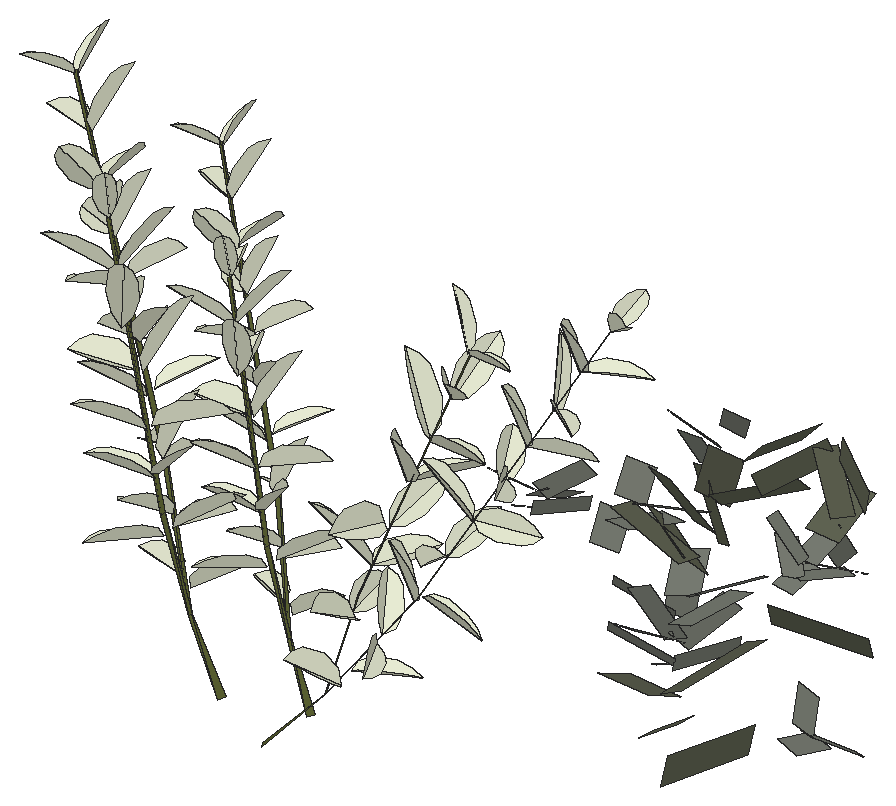
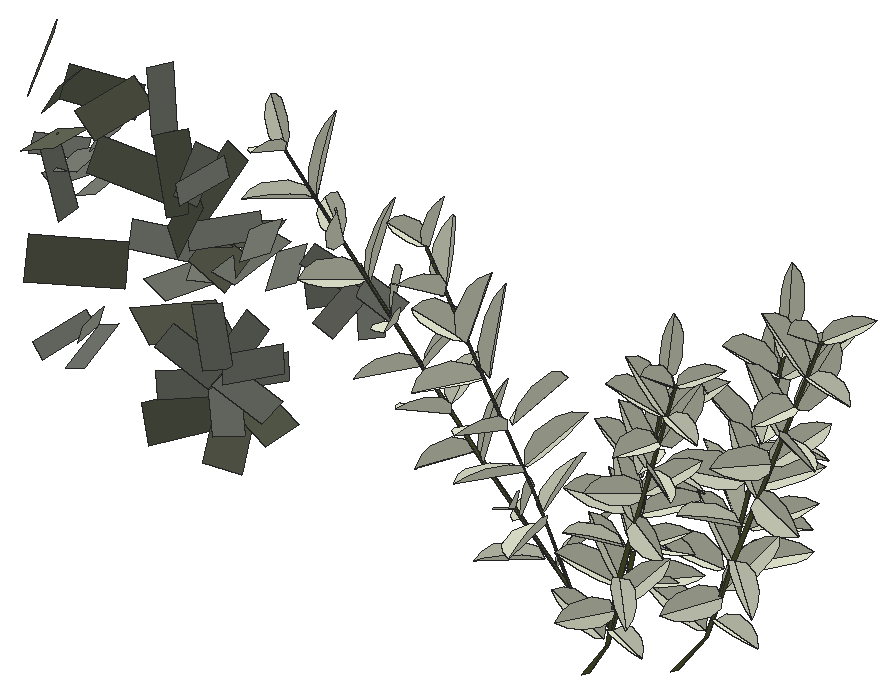
# SketchUp Ruby script. Lengths in inches.
U = 1.inch
M = Sketchup.active_model
def pt(a) = Geom::Point3d.new(a.map { |v| v * U })
def face(e, loops, mat)
  f = e.add_face(loops[0].map { |a| pt(a) })
  loops[1..].each { |l| e.add_face(l.map { |a| pt(a) }).erase! }
  f.material = f.back_material = mat if mat
  f
end
# faces: each face lists its corners as indices into pts; further lists are holes
def faces(e, pts, list, mat = nil) = list.each { |f| face(e, (f[0].is_a?(Array) ? f : [f]).map { |l| l.map { |i| pts[i] } }, mat) }
# xy, xz, yz: faces in a plane at the given z, y or x. An outline is a flat list of corners, or four numbers for a rectangle; further outlines are holes
def ring(l) = l.size == 4 ? [[l[0], l[1]], [l[2], l[1]], [l[2], l[3]], [l[0], l[3]]] : l.each_slice(2).to_a
def flat(e, list, mat, &to3) = list.each { |f| face(e, (f[0].is_a?(Array) ? f : [f]).map { |l| ring(l).map { |u, v| to3.(u, v) } }, mat) }
def xy(e, z, list, mat = nil) = flat(e, list, mat) { |x, y| [x, y, z] }
def xz(e, y, list, mat = nil) = flat(e, list, mat) { |x, z| [x, y, z] }
def yz(e, x, list, mat = nil) = flat(e, list, mat) { |y, z| [x, y, z] }
def lines(e, pts, list) = list.each { |a, b| e.add_line(pt(pts[a]), pt(pts[b])) }
# prism: a flat outline (further loops are holes) pulled along v
def prism(e, loops, v, mat = nil)
  f = face(e, loops, mat); d = Geom::Vector3d.new(v.map { |x| x * U })
  f.pushpull(f.normal.samedirection?(d) ? d.length : -d.length)
end
def box(e, o, s, mat = nil) = prism(e, [[o, [o[0] + s[0], o[1], o[2]], [o[0] + s[0], o[1] + s[1], o[2]], [o[0], o[1] + s[1], o[2]]]], [0, 0, s[2]], mat)
def at(x, y, z, deg = 0) = Geom::Transformation.translation(pt([x, y, z])) * Geom::Transformation.rotation(ORIGIN, Z_AXIS, deg.degrees)
def axes(o, x, y, z) = Geom::Transformation.new([*x, 0, *y, 0, *z, 0, *pt(o).to_a, 1])
def part(name) = M.definitions.add(name)
# library, detail: a bought-in or finely detailed component or shape, given as its bounding box
def library(name, o, s) = part(name).tap { |d| box(d.entities, o, s) }
def detail(e, o, s) = box(e.add_group.entities, o, s)
def put(e, d, t, mat = nil) = e.add_instance(d, t).tap { |i| i.material = mat if mat }
def group(e, t, mat = nil) = e.add_group.tap { |g| g.transformation = t; g.material = mat if mat }.entities
root = M.entities
M.materials.add("asdfasdf0165f6asdLeafVar1sfd015as60f1as6").color = [231, 235, 211]
M.materials.add("dw_stemssadfasdfa0sdf1s01d6w1").color = [90, 97, 50]
M.materials.add("viburnumblaasdfas0df1w06d").color = [98, 102, 84]
M.materials.add("viburnumbladsadfasdfad0w122").color = [125, 129, 119]
c1 = part("Component\#314")
p = [[0.14,0,0],[2.58,0.05,0.25],[2.44,5.11,2.64],[0,5.05,2.39]]
faces(c1.entities,p,[[0,1,2,3]],"viburnumblaasdfas0df1w06d")
c2 = part("viburnumblad1\#2")
put(c2.entities,c1,axes([-37.25,6.23,19.31],[75.98784,0,0],[0,65.50676,0],[0,0,75.98784]))
c3 = part("Component\#315")
p = [[0.25,0,0],[2.05,0.01,0.35],[1.81,4.2,1.66],[0,4.19,1.3125]]
faces(c3.entities,p,[[0,1,2,3]],"viburnumbladsadfasdfad0w122")
c4 = part("viburnumblad2")
put(c4.entities,c3,axes([-19.23,-4.49,-32.18],[83.35428,0,0],[0,79.38502,0],[0,0,83.35428]))
c5 = part("vdw_leaf\#3")
p = [[0,0,0],[-2.77,1.61,2.32],[-4.3125,6.1,4.5],[-3.97,13.49,6.09],[-2.47,18.57,6.3],[-0.2,22.73,5.75],
  [2.54,19.66,6.85],[4.3,15.93,7.09],[5.03,7.6,5.43],[3.32,1.76,2.74]]
faces(c5.entities,p,[[0,1,2,3,4,5],[0,5,6,7,8,9]],"asdfasdf0165f6asdLeafVar1sfd015as60f1as6")
c6 = part("dw_brancj_2\#2")
p = [[9.7,-0.22,29.95],[0.23,-1.96,0.34],[-0.05,1.51,0.11],[9.65,1.51,29.46],[18.64,-8.75,84.43],[18.96,-6.63,84.625],
  [1.53,6.02,63.68],[1.42,8.18,63.25],[-10.58,8.77,161.17],[-10.41,9.98,160.68],[26.34,-9.37,211.72],[26.57,-8.28,211.23]]
faces(c6.entities,p,[[0,1,2],[0,2,3],[4,0,3],[4,3,5],[6,0,3],[6,3,7],[8,6,7],[8,7,9],
  [10,4,5],[10,5,11]],"dw_stemssadfasdfa0sdf1s01d6w1")
c7 = part("vdw_branch2\#3")
put(c7.entities,c5,axes([19.53,-5.9,102.42],[1.12377,-0.50004,0],[0.46097,1.03596,0.47664],[-0.19377,-0.43548,1.13389]))
put(c7.entities,c5,axes([-5.89,6.52,109.44],[-1.07209,0.83679,0],[-0.77141,-0.98832,0.52702],[0.32427,0.41545,1.25373]))
put(c7.entities,c5,axes([-0.44,8.23,75.28],[0.88709,-0.9947,0],[0.92159,0.82189,0.33087],[-0.25219,-0.22491,1.26111]))
put(c7.entities,c5,axes([24.71,-8.97,190.81],[-0.82641,0.91101,0],[-0.83983,-0.76184,0.47664],[0.35303,0.32025,1.13389]))
put(c7.entities,c5,axes([-2.29,8.24,91.35],[1.24603,-0.47303,0],[0.43826,1.15445,0.33087],[-0.11993,-0.31592,1.26111]))
put(c7.entities,c5,axes([12.26,-3.11,37.92],[-0.64625,1.02205,0.22511],[-1.04383,-0.61044,-0.22511],[-0.07533,-0.30931,1.18809]))
put(c7.entities,c5,axes([26.17,-9.17,210.27],[-0.99452,-0.10453,0],[0.09636,-0.91681,0.38752],[-0.04051,0.38539,0.92186]))
put(c7.entities,c5,axes([-6.07,9.4,125.35],[-0.90214,-0.98107,0],[0.90896,-0.83583,0.33087],[-0.24874,0.22873,1.26111]))
put(c7.entities,c5,axes([-4.13,7.29,110.58],[0.44715,-1.078,0.64369],[1.05816,0.63649,0.33087],[-0.58725,0.40856,1.09216]))
put(c7.entities,c5,axes([23.91,-8.22,171.96],[0.62307,0.85009,-0.63406],[-0.71531,0.8798,0.47664],[0.78296,0.12729,0.94004]))
put(c7.entities,c6,at(-0.09,0.18,-0.25),"dw_stemssadfasdfa0sdf1s01d6w1")
put(c7.entities,c5,axes([23.34,-9.65,156.59],[-0.31364,-1.00782,0.58216],[1.10369,-0.17062,0.29925],[-0.17137,0.6239,0.98776]))
put(c7.entities,c5,axes([15.03,-3.37,58.83],[-1.05425,-0.00194,0.58442],[-0.14303,-1.11707,-0.26172],[0.55355,-0.3046,0.99755]))
put(c7.entities,c5,axes([-11.625,9.46,160.37],[0.36812,0.92978,0],[-0.85713,0.33936,0.38752],[0.3603,-0.14265,0.92186]))
put(c7.entities,c5,axes([21.32,-8.53,138.72],[1.21379,0.19904,0],[-0.19904,1.21379,0],[0,0,1.23]))
put(c7.entities,c5,axes([22.54,-9.2,141.43],[-1.02887,0.17955,0.60182],[-0.23387,-1.13057,-0.06253],[0.56696,-0.17376,1.02111]))
put(c7.entities,c5,axes([23.9,-8.82,173.84],[-1.14567,-0.37474,0],[0.35918,-1.0981,0.04438],[-0.01409,0.04308,1.17993]))
put(c7.entities,c5,axes([-7.84,8.92,143.59],[-1.26971,0.40522,0],[-0.37543,-1.17638,0.33087],[0.10274,0.32192,1.26111]))
put(c7.entities,c5,axes([19.77,-8.01,85.98],[-0.32405,-1.14591,0.18674],[1.10278,-0.32969,-0.10948],[0.15845,0.14442,1.16117]))
put(c7.entities,c5,axes([-0.62,5.76,76.34],[-0.08879,1.17576,-0.67771],[-1.34525,-0.16582,-0.11144],[-0.17897,0.66309,1.17383]))
put(c7.entities,c5,axes([20.49,-8.22,121.07],[0.39924,-0.78471,-0.8233],[1.08735,0.33121,0.2116],[0.09035,-0.83005,0.83495]))
put(c7.entities,c5,axes([15.15,-3.72,62.9],[1.16251,0.40128,-0.0211],[-0.39924,1.16074,0.07874],[0.0456,-0.06757,1.2273]))
put(c7.entities,c5,axes([20.72,-8.08,120.26],[-0.03693,1.2277,-0.06551],[-1.22944,-0.03698,0],[-0.00197,0.06548,1.22825]))
put(c7.entities,c5,axes([22.58,-8.36,155.57],[-0.56247,1.09386,0],[-1.00839,-0.51852,0.47664],[0.42389,0.21796,1.13389]))
put(c7.entities,c5,axes([3.97,3.13,57.96],[-1.09459,0.76041,0],[-0.72262,-1.0402,-0.1735],[-0.10109,-0.14552,1.29352]))
put(c7.entities,c5,axes([-10.8,9.06,160.75],[-0.66334,-0.72138,0],[0.66835,-0.61458,0.24329],[-0.1829,0.16818,0.92729]))
put(c7.entities,c5,axes([19.06,-9.3125,103.96],[-1.01345,0.25553,-0.60051],[-0.2265,-1.12952,-0.09839],[-0.59598,0.03076,1.01889]))
put(c7.entities,c5,axes([18.07,-6.2,81.7],[-0.56247,1.09386,0],[-1.00839,-0.51852,0.47664],[0.42389,0.21796,1.13389]))
put(c7.entities,c5,axes([12.95,-0.39,43.31],[0.13044,-1.19832,0],[1.11025,0.12085,0.29925],[-0.30382,-0.03307,1.14057]))
put(c7.entities,c5,axes([2.28,8.28,56.18],[1.32413,-0.31027,0],[0.30923,1.31968,-0.11144],[0.02542,0.1085,1.35543]))
put(c7.entities,c5,axes([-7.55,9.96,143.07],[1.34251,-0.21744,0],[0.20045,1.23761,0.52702],[-0.08426,-0.52024,1.25373]))
put(c7.entities,c5,axes([26.15,-8.25,210.66],[0.94661,-0.25364,0],[0.235,0.87703,0.24329],[-0.06431,-0.24,0.92729]))
put(c7.entities,c5,axes([-6.48,11.37,125.16],[0.64635,1.10315,0.46356],[-1.16569,0.46153,0.52702],[0.27017,-0.6478,1.16488]))
put(c7.entities,c5,axes([25.74,-8.35,191.28],[0.13044,-1.19832,0],[1.11025,0.12085,0.29925],[-0.30382,-0.03307,1.14057]))
put(c7.entities,c5,axes([-5.125,7.47,91.6],[-1.10024,0.63688,0.48318],[-0.78682,-1.00808,-0.46292],[0.14137,-0.65404,1.184]))
put(root,c2,axes([1229.8,292.03,5.5],[0.00521,-0.00318,0.0136],[0.01189,0.01244,-0.00164],[-0.00949,0.00985,0.00593]))
put(root,c4,axes([1238.96,294.58,23.71],[-0.00315,0.00923,-0.0035],[-0.009,-0.00109,0.00491],[0.00408,0.00455,0.00739]))
put(root,c2,axes([1229.78,294.23,20.15],[-0.00128,0.01292,-0.00526],[-0.01614,-0.0018,-0.00049],[-0.00098,0.00473,0.0118]))
put(root,c2,axes([1229.76,292.29,11.59],[0.01313,-0.00582,0.00636],[0.00841,0.01593,-0.00278],[-0.00467,0.00494,0.01417]))
put(root,c4,axes([1223.64,293.02,20.79],[0.00973,0.00497,-0.00674],[-0.00836,0.01112,-0.00387],[0.00402,0.00678,0.0108]))
put(root,c7,axes([1195,291.84,-0.375],[-0.13136,0.05263,-0.10053],[-0.06077,-0.15168,0],[-0.07584,0.03038,0.17413]))
put(root,c4,axes([1216.74,293.95,20.41],[0.00898,0.00541,-0.00233],[-0.00533,0.00547,-0.00762],[-0.00249,0.00719,0.00626]))
put(root,c2,axes([1230.42,296.33,21.7],[-0.01202,0.00402,-0.00269],[-0.00561,-0.01134,0.00795],[0.00019,0.00723,0.00942]))
put(root,c7,axes([1199.63,290.12,-1.28],[0.12089,0.06455,-0.10951],[-0.07696,0.14414,0],[0.0785,0.04192,0.16863]))
put(root,c4,axes([1216.89,294.82,21.52],[0.00286,0.007,-0.00749],[-0.01015,0.00031,-0.00351],[-0.0019,0.00782,0.00576]))
put(root,c4,axes([1238.02,294.15,22.79],[0.00444,0.00768,-0.00528],[-0.00777,0.00538,0.00119],[0.00402,0.0037,0.00783]))
put(root,c2,axes([1227.75,293.87,10.14],[0.00536,0.01158,-0.00521],[-0.01304,0.00197,-0.00903],[-0.0059,0.00728,0.01011]))
put(root,c4,axes([1229.72,295.18,18.16],[0.00715,-0.01146,0.00475],[0.01219,0.00751,-0.00024],[-0.0023,0.00416,0.01351]))
put(root,c4,axes([1217.29,294.85,19.55],[0.00494,-0.0045,0.00826],[0.00853,0.00632,-0.00167],[-0.00419,0.00708,0.00554]))
put(root,c2,axes([1227.99,292.7,7.87],[0.01075,0.00741,0.00439],[-0.00265,0.0107,-0.01157],[-0.00831,0.00706,0.00843]))
put(root,c4,axes([1229.23,293.68,16.72],[0.01381,-0.0032,0.00202],[0.00375,0.01421,-0.00318],[-0.00124,0.00342,0.01385]))
put(root,c4,axes([1227.42,296.46,12.26],[-0.00484,0.0048,-0.00995],[-0.01148,-0.00686,0.00228],[-0.0044,0.00962,0.00678]))
put(root,c4,axes([1237.17,294.3,21.79],[0.00829,0.00118,-0.00446],[-0.00277,0.00969,-0.0025],[0.00431,0.00339,0.00782]))
put(root,c4,axes([1238.6875,296.25,22.97],[0.00315,-0.00923,0.0035],[0.00972,0.00216,-0.00297],[0.00178,0.00415,0.00836]))
put(root,c4,axes([1237.5,294.51,10.76],[0.00948,-0.00167,-0.00544],[-0.00216,0.00929,-0.00661],[0.00531,0.00641,0.00728]))
put(root,c4,axes([1217.69,296.07,20.33],[-0.00286,-0.007,0.00749],[0.00939,0.00159,0.0048],[-0.00429,0.00766,0.00474]))
put(root,c4,axes([1228.96,293.63,18.7],[0.01238,0.00695,-0.00189],[-0.0072,0.01199,-0.00308],[0.00008,0.00361,0.01386]))
put(root,c4,axes([1237.59,295.47,22.32],[0.00889,-0.00537,-0.00033],[0.00481,0.00824,-0.00432],[0.00239,0.00342,0.00851]))
put(root,c4,axes([1223.65,294.65,21.63],[0.01295,-0.00298,-0.00152],[0.00183,0.01176,-0.00745],[0.00286,0.00667,0.01124]))
put(root,c4,axes([1238.18,296,10.96],[0.0086,-0.00684,0.0012],[0.00538,0.00535,-0.00804],[0.0044,0.00684,0.00749]))
put(root,c4,axes([1238.31,295.04,11.96],[0.0048,0.00448,-0.0089],[-0.00793,0.0077,-0.0004],[0.00603,0.00655,0.00655]))
put(root,c2,axes([1235.11,295.17,26.65],[0.00085,-0.00676,0.01003],[0.01236,0.00601,0.00299],[-0.00572,0.00864,0.0063]))
put(root,c4,axes([1227.2,297.95,13],[-0.01065,-0.00175,-0.00643],[-0.00418,-0.00769,0.00902],[-0.00519,0.00978,0.00593]))
put(root,c4,axes([1224.45,296.34,22.32],[0.00818,-0.0094,0.00487],[0.01043,0.00611,-0.00572],[0.00179,0.0073,0.01107]))
put(root,c4,axes([1231.33,298.72,28.41],[-0.00994,-0.00547,0.00222],[0.00636,-0.00933,0.00551],[-0.00082,0.00596,0.01103]))
put(root,c2,axes([1241.92,297.13,26.98],[-0.00677,0.00906,0.00107],[-0.00671,-0.00636,0.00903],[0.00707,0.00408,0.0069]))
put(root,c2,axes([1229.54,294.79,20.07],[0.00337,0.00858,-0.01052],[-0.01574,0.00327,-0.00237],[0.0008,0.00999,0.00793]))
put(root,c4,axes([1216.47,295.5,20.44],[0.00984,0.00064,0.00419],[0.00246,0.0079,-0.00679],[-0.00344,0.00689,0.00616]))
put(root,c4,axes([1237.94,295.41,23.64],[0.00943,0.00164,-0.00397],[-0.00277,0.00969,-0.0025],[0.00332,0.00323,0.0083]))
put(root,c4,axes([1224,295.12,23.4],[0.01014,0.00518,-0.00703],[-0.00774,0.0103,-0.00358],[0.00402,0.00678,0.0108]))
put(root,c2,axes([1229.72,298.37,22.52],[-0.01137,-0.00525,0.00325],[0.00699,-0.00886,0.00961],[-0.00151,0.00884,0.00798]))
put(root,c2,axes([1240.32,296.03,26.31],[0.00134,0.01062,-0.0039],[-0.01115,0.00362,0.00577],[0.00594,0.00252,0.00833]))
put(root,c4,axes([1226.03,297.13,13.03],[0.00352,0.00882,-0.00823],[-0.01182,-0.0007,-0.00581],[-0.00432,0.00892,0.00772]))
put(root,c4,axes([1225.88,298.38,14.25],[-0.00504,0.005,-0.01036],[-0.01063,-0.00635,0.00211],[-0.0044,0.00962,0.00678]))
put(root,c2,axes([1230.89,297.1,20.58],[-0.00982,0.00575,-0.00616],[-0.00925,-0.00382,0.01097],[0.00277,0.01054,0.00496]))
put(root,c4,axes([1226.09,296.36,11.375],[0.01046,0.00781,-0.00132],[-0.00513,0.00543,-0.00849],[-0.00501,0.0081,0.0082]))
put(root,c2,axes([1233.82,297.51,16.09],[0.0041,-0.00986,0.01208],[0.01717,-0.00172,-0.00723],[0.00492,0.01267,0.00868]))
put(root,c4,axes([1229.02,299.35,25.03],[-0.01201,-0.00131,-0.00224],[-0.00042,-0.0083,0.00649],[-0.00262,0.00705,0.00788]))
put(root,c2,axes([1230.02,297.41,23.09],[0.00221,-0.01095,0.00807],[0.01572,0.00285,-0.00044],[-0.00114,0.008,0.01116]))
put(root,c2,axes([1233.66,295.63,28.32],[0.00897,-0.0006,0.00814],[0.00562,0.01175,-0.00532],[-0.00657,0.00665,0.00773]))
put(root,c4,axes([1226.56,297.39,10.64],[0.00529,-0.00535,0.00878],[0.00925,0.00849,-0.00041],[-0.00626,0.00721,0.00817]))
put(root,c4,axes([1226.55,299.51,13.37],[-0.01002,-0.00748,0.00127],[0.00432,-0.00389,0.01114],[-0.00624,0.00932,0.00567]))
put(root,c2,axes([1238.4375,295.95,24.83],[0.01113,0.00289,-0.00438],[-0.00454,0.01328,-0.00273],[0.00348,0.00335,0.01016]))
put(root,c4,axes([1237.75,300.29,20.6],[-0.0106,-0.00225,0.00809],[0.00771,-0.01018,0.00728],[0.00487,0.01032,0.00927]))
put(root,c4,axes([1226.75,298.72,11.66],[-0.00352,-0.00882,0.00823],[0.00998,0.00284,0.00731],[-0.00692,0.00849,0.00615]))
put(root,c7,axes([1199.9,294.57,-1.1],[-0.10999,0.0642,-0.09048],[-0.07413,-0.12701,0],[-0.0635,0.03707,0.15671]))
put(root,c4,axes([1228.57,299.67,26.24],[-0.00804,0.00619,-0.0059],[-0.0078,-0.0066,0.00358],[-0.00163,0.0068,0.00829]))
